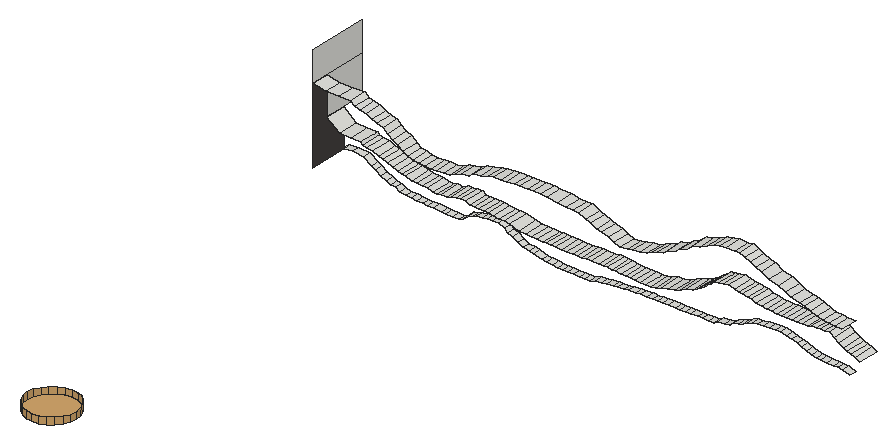
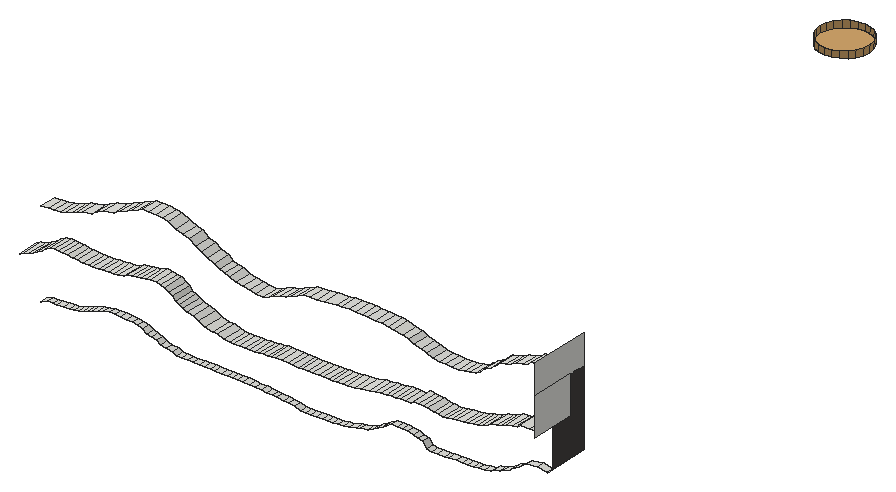
# SketchUp Ruby script. Lengths in inches.
U = 1.inch
M = Sketchup.active_model
def pt(a) = Geom::Point3d.new(a.map { |v| v * U })
def face(e, loops, mat)
  f = e.add_face(loops[0].map { |a| pt(a) })
  loops[1..].each { |l| e.add_face(l.map { |a| pt(a) }).erase! }
  f.material = f.back_material = mat if mat
  f
end
# faces: each face lists its corners as indices into pts; further lists are holes
def faces(e, pts, list, mat = nil) = list.each { |f| face(e, (f[0].is_a?(Array) ? f : [f]).map { |l| l.map { |i| pts[i] } }, mat) }
# xy, xz, yz: faces in a plane at the given z, y or x. An outline is a flat list of corners, or four numbers for a rectangle; further outlines are holes
def ring(l) = l.size == 4 ? [[l[0], l[1]], [l[2], l[1]], [l[2], l[3]], [l[0], l[3]]] : l.each_slice(2).to_a
def flat(e, list, mat, &to3) = list.each { |f| face(e, (f[0].is_a?(Array) ? f : [f]).map { |l| ring(l).map { |u, v| to3.(u, v) } }, mat) }
def xy(e, z, list, mat = nil) = flat(e, list, mat) { |x, y| [x, y, z] }
def xz(e, y, list, mat = nil) = flat(e, list, mat) { |x, z| [x, y, z] }
def yz(e, x, list, mat = nil) = flat(e, list, mat) { |y, z| [x, y, z] }
def lines(e, pts, list) = list.each { |a, b| e.add_line(pt(pts[a]), pt(pts[b])) }
# prism: a flat outline (further loops are holes) pulled along v
def prism(e, loops, v, mat = nil)
  f = face(e, loops, mat); d = Geom::Vector3d.new(v.map { |x| x * U })
  f.pushpull(f.normal.samedirection?(d) ? d.length : -d.length)
end
def box(e, o, s, mat = nil) = prism(e, [[o, [o[0] + s[0], o[1], o[2]], [o[0] + s[0], o[1] + s[1], o[2]], [o[0], o[1] + s[1], o[2]]]], [0, 0, s[2]], mat)
def at(x, y, z, deg = 0) = Geom::Transformation.translation(pt([x, y, z])) * Geom::Transformation.rotation(ORIGIN, Z_AXIS, deg.degrees)
def axes(o, x, y, z) = Geom::Transformation.new([*x, 0, *y, 0, *z, 0, *pt(o).to_a, 1])
def part(name) = M.definitions.add(name)
# library, detail: a bought-in or finely detailed component or shape, given as its bounding box
def library(name, o, s) = part(name).tap { |d| box(d.entities, o, s) }
def detail(e, o, s) = box(e.add_group.entities, o, s)
def put(e, d, t, mat = nil) = e.add_instance(d, t).tap { |i| i.material = mat if mat }
def group(e, t, mat = nil) = e.add_group.tap { |g| g.transformation = t; g.material = mat if mat }.entities
root = M.entities
M.materials.add("[Field Square Tile]").color = [211, 167, 108]
M.materials.add("[Granite Tile]1").color = [68, 65, 63]
xy(root,237.65,[[2918.33,2401.37,2919.02,2402.3],[2919.02,2401.37,2919.64,2402.3]])
xy(root,238.33,[[2927.43,2401.37,2927.98,2402.3],[2927.98,2401.37,2928.66,2402.3]])
xy(root,238.34,[[2929.34,2401.37,2930.27,2402.3],[2930.27,2401.37,2930.76,2402.3],[2930.76,2401.37,2931.52,2402.3],[2931.52,2401.37,2932.15,2402.3],[2932.15,2401.37,2932.9,2402.3],
  [2932.9,2401.37,2933.52,2402.3],[2933.52,2401.37,2934.29,2402.3],[2934.29,2401.37,2934.91,2402.3]])
xy(root,241.52,[[2889.03,2396.68,2889.09,2402.3]])
xy(root,241.68,[[2919.53,2398.8,2920.12,2401.37]])
xy(root,241.75,[[2921.88,2398.8,2922.75,2401.37],[2922.75,2398.8,2923.37,2401.37],[2923.37,2398.8,2923.88,2401.37]])
xy(root,250.6875,[[2909.35,2327.89,2908.56,2328,2907.82,2328.3,2907.18,2328.79,2906.7,2329.43,2906.39,2330.16,2906.29,2330.96,2906.39,2331.75,2906.7,2332.49,2907.18,2333.12,2907.82,2333.61,2908.56,2333.91,2909.35,2334.02,2910.14,2333.91,2910.88,2333.61,2911.51,2333.12,2912,2332.49,2912.31,2331.75,2912.41,2330.96,2912.31,2330.16,2912,2329.43,2911.51,2328.79,2910.88,2328.3,2910.14,2328]],"[Field Square Tile]")
xz(root,2396.68,[[2889.03,241.52,2889.09,251.5]])
yz(root,2889.09,[[2398.8,246.2,2404.3,250.88],[2396.68,250.88,2404.3,254.5]])
yz(root,2889.09,[[2396.68,241.52,2401.37,241.52,2401.37,246.2,2398.8,246.2,2398.8,250.88,2396.68,250.88]],"[Granite Tile]1")
p = [[2919.64,2401.37,237.65],[2919.64,2402.3,237.65],[2920.31,2402.3,237.89],[2920.31,2401.37,237.89],[2914.97,2401.37,237.76],[2914.97,2402.3,237.76],
  [2915.68,2402.3,237.71],[2915.68,2401.37,237.71],[2916.29,2402.3,237.68],[2916.29,2401.37,237.68],[2916.89,2402.3,237.67],[2916.89,2401.37,237.67],
  [2917.64,2402.3,237.66],[2917.64,2401.37,237.66],[2918.33,2402.3,237.65],[2918.33,2401.37,237.65],[2913.62,2401.37,237.9],[2913.62,2402.3,237.9],
  [2914.28,2402.3,237.82],[2914.28,2401.37,237.82],[2912.68,2401.37,238.21],[2912.68,2402.3,238.21],[2921.07,2402.3,237.94],[2921.07,2401.37,237.94],
  [2921.6875,2402.3,237.98],[2921.6875,2401.37,237.98],[2922.54,2402.3,238.1],[2922.54,2401.37,238.1],[2923.09,2402.3,238.13],[2923.09,2401.37,238.13],
  [2923.85,2402.3,238.15],[2923.85,2401.37,238.15],[2912.21,2401.37,238.31],[2912.21,2402.3,238.31],[2924.48,2402.3,238.26],[2924.48,2401.37,238.26],
  [2911.3,2401.37,238.43],[2911.3,2402.3,238.43],[2925.23,2402.3,238.28],[2925.23,2401.37,238.28],[2925.86,2402.3,238.3],[2925.86,2401.37,238.3],
  [2926.71,2402.3,238.32],[2926.71,2401.37,238.32],[2927.43,2402.3,238.33],[2927.43,2401.37,238.33],[2928.66,2401.37,238.33],[2928.66,2402.3,238.33],
  [2929.34,2402.3,238.34],[2929.34,2401.37,238.34],[2934.91,2401.37,238.34],[2934.91,2402.3,238.34],[2935.42,2402.3,238.59],[2935.42,2401.37,238.59],
  [2910.65,2401.37,238.74],[2910.65,2402.3,238.74],[2950.94,2401.37,238.78],[2950.94,2402.3,238.78],[2951.72,2402.3,238.43],[2951.72,2401.37,238.43],
  [2936.24,2402.3,238.72],[2936.24,2401.37,238.72],[2910.07,2401.37,239.11],[2910.07,2402.3,239.11],[2936.93,2402.3,238.86],[2936.93,2401.37,238.86],
  [2900.28,2401.37,238.92],[2900.28,2402.3,238.92],[2901.32,2402.3,238.82],[2901.32,2401.37,238.82],[2901.83,2402.3,238.8],[2901.83,2401.37,238.8],
  [2902.7,2402.3,238.79],[2902.7,2401.37,238.79],[2903.44,2402.3,238.77],[2903.44,2401.37,238.77],[2903.97,2402.3,238.9375],[2903.97,2401.37,238.9375],
  [2948.22,2401.37,238.875],[2948.22,2402.3,238.875],[2948.97,2402.3,238.83],[2948.97,2401.37,238.83],[2949.73,2402.3,238.8],[2949.73,2401.37,238.8],
  [2950.27,2402.3,238.79],[2950.27,2401.37,238.79],[2898.19,2401.37,238.97],[2898.19,2402.3,238.97],[2898.89,2402.3,238.94],[2898.89,2401.37,238.94],
  [2899.59,2402.3,238.93],[2899.59,2401.37,238.93],[2904.53,2402.3,239.55],[2904.53,2401.37,239.55],[2937.44,2402.3,239.18],[2937.44,2401.37,239.18],
  [2947.07,2401.37,239.04],[2947.07,2402.3,239.04],[2947.65,2402.3,238.94],[2947.65,2401.37,238.94],[2896.82,2401.37,239.09],[2896.82,2402.3,239.09],
  [2897.51,2402.3,239.03],[2897.51,2401.37,239.03],[2946.41,2401.37,239.29],[2946.41,2402.3,239.29],[2896.04,2401.37,239.19],[2896.04,2402.3,239.19],
  [2909.49,2401.37,239.38],[2909.49,2402.3,239.38],[2895.53,2401.37,239.52],[2895.53,2402.3,239.52],[2938.03,2402.3,239.35],[2938.03,2401.37,239.35],
  [2945.83,2401.37,239.53],[2945.83,2402.3,239.53],[2909.03,2401.37,239.71],[2909.03,2402.3,239.71],[2938.59,2402.3,239.52],[2938.59,2401.37,239.52],
  [2894.97,2401.37,239.64],[2894.97,2402.3,239.64],[2939.14,2402.3,239.85],[2939.14,2401.37,239.85],[2945.3,2401.37,239.7],[2945.3,2402.3,239.7],
  [2894.52,2401.37,239.86],[2894.52,2402.3,239.86],[2905.11,2402.3,239.69],[2905.11,2401.37,239.69],[2905.66,2402.3,239.88],[2905.66,2401.37,239.88],
  [2908.33,2401.37,240.11],[2908.33,2402.3,240.11],[2944.61,2401.37,239.92],[2944.61,2402.3,239.92],[2939.78,2402.3,240.03],[2939.78,2401.37,240.03],
  [2893.73,2401.37,240.2],[2893.73,2402.3,240.2],[2906.39,2402.3,239.99],[2906.39,2401.37,239.99],[2943.98,2401.37,240.11],[2943.98,2402.3,240.11],
  [2906.98,2402.3,240.05],[2906.98,2401.37,240.05],[2907.64,2402.3,240.09],[2907.64,2401.37,240.09],[2940.4375,2402.3,240.12],[2940.4375,2401.37,240.12],
  [2941.11,2402.3,240.19],[2941.11,2401.37,240.19],[2943.2,2401.37,240.27],[2943.2,2402.3,240.27],[2893.13,2401.37,240.59],[2893.13,2402.3,240.59],
  [2941.875,2402.3,240.23],[2941.875,2401.37,240.23],[2942.58,2402.3,240.25],[2942.58,2401.37,240.25],[2892.59,2401.37,240.85],[2892.59,2402.3,240.85],
  [2891.57,2401.37,241.55],[2891.57,2402.3,241.55],[2925.51,2398.8,241.57],[2925.51,2401.37,241.57],[2926.05,2401.37,241.53],[2926.05,2398.8,241.53],
  [2926.67,2401.37,241.51],[2926.67,2398.8,241.51],[2927.22,2401.37,241.49],[2927.22,2398.8,241.49],[2927.92,2401.37,241.48],[2927.92,2398.8,241.48],
  [2928.58,2401.37,241.47],[2928.58,2398.8,241.47],[2929.15,2401.37,241.46],[2929.15,2398.8,241.46],[2929.86,2401.37,241.6],[2929.86,2398.8,241.6],
  [2889.09,2401.37,241.52],[2889.09,2402.3,241.52],[2890.3,2402.3,241.69],[2890.3,2401.37,241.69],[2924.9,2398.8,241.66],[2924.9,2401.37,241.66],
  [2930.59,2401.37,241.85],[2930.59,2398.8,241.85],[2915.87,2398.8,241.75],[2915.87,2401.37,241.75],[2916.32,2401.37,241.74],[2916.32,2398.8,241.74],
  [2916.87,2401.37,241.72],[2916.87,2398.8,241.72],[2917.5,2401.37,241.71],[2917.5,2398.8,241.71],[2918.13,2401.37,241.7],[2918.13,2398.8,241.7],
  [2918.86,2401.37,241.69],[2918.86,2398.8,241.69],[2919.53,2401.37,241.68],[2919.53,2398.8,241.68],[2920.12,2398.8,241.68],[2920.12,2401.37,241.68],
  [2920.61,2401.37,241.67],[2920.61,2398.8,241.67],[2921.3125,2401.37,241.74],[2921.3125,2398.8,241.74],[2921.88,2401.37,241.75],[2921.88,2398.8,241.75],
  [2923.88,2398.8,241.75],[2923.88,2401.37,241.75],[2924.37,2401.37,241.67],[2924.37,2398.8,241.67],[2913.68,2398.8,241.89],[2913.68,2401.37,241.89],
  [2914.5,2401.37,241.83],[2914.5,2398.8,241.83],[2915.1,2401.37,241.78],[2915.1,2398.8,241.78],[2931.26,2401.37,241.91],[2931.26,2398.8,241.91],
  [2912.91,2398.8,241.96],[2912.91,2401.37,241.96],[2932.16,2401.37,242.1],[2932.16,2398.8,242.1],[2911.74,2398.8,242.24],[2911.74,2401.37,242.24],
  [2932.93,2401.37,242.46],[2932.93,2398.8,242.46],[2911.07,2398.8,242.34],[2911.07,2401.37,242.34],[2954.54,2398.8,242.51],[2954.54,2401.37,242.51],
  [2955.05,2401.37,242.21],[2955.05,2398.8,242.21],[2910.41,2398.8,242.38],[2910.41,2401.37,242.38],[2909.75,2398.8,242.48],[2909.75,2401.37,242.48],
  [2901.57,2398.8,242.68],[2901.57,2401.37,242.68],[2902.24,2401.37,242.51],[2902.24,2398.8,242.51],[2902.76,2401.37,242.46],[2902.76,2398.8,242.46],
  [2903.3,2401.37,242.58],[2903.3,2398.8,242.58],[2909.11,2398.8,242.57],[2909.11,2401.37,242.57],[2933.63,2401.37,242.78],[2933.63,2398.8,242.78],
  [2953.95,2398.8,242.68],[2953.95,2401.37,242.68],[2903.93,2401.37,242.57],[2903.93,2398.8,242.57],[2904.56,2401.37,242.81],[2904.56,2398.8,242.81],
  [2906.33,2398.8,242.92],[2906.33,2401.37,242.92],[2906.76,2401.37,242.625],[2906.76,2398.8,242.625],[2907.37,2401.37,242.65],[2907.37,2398.8,242.65],
  [2907.92,2401.37,242.62],[2907.92,2398.8,242.62],[2908.55,2401.37,242.58],[2908.55,2398.8,242.58],[2900.22,2398.8,242.78],[2900.22,2401.37,242.78],
  [2901.03,2401.37,242.73],[2901.03,2398.8,242.73],[2953.45,2398.8,242.875],[2953.45,2401.37,242.875],[2898.92,2398.8,243.06],[2898.92,2401.37,243.06],
  [2899.64,2401.37,242.85],[2899.64,2398.8,242.85],[2905.13,2401.37,242.86],[2905.13,2398.8,242.86],[2934.4,2401.37,242.97],[2934.4,2398.8,242.97],
  [2905.69,2401.37,242.89],[2905.69,2398.8,242.89],[2953.06,2398.8,243.09],[2953.06,2401.37,243.09],[2934.93,2401.37,243.23],[2934.93,2398.8,243.23],
  [2897.85,2398.8,243.3],[2897.85,2401.37,243.3],[2898.4375,2401.37,243.14],[2898.4375,2398.8,243.14],[2952.45,2398.8,243.43],[2952.45,2401.37,243.43],
  [2935.33,2401.37,243.48],[2935.33,2398.8,243.48],[2897.21,2398.8,243.48],[2897.21,2401.37,243.48],[2951.91,2398.8,243.8],[2951.91,2401.37,243.8],
  [2896.69,2398.8,243.79],[2896.69,2401.37,243.79],[2935.85,2401.37,243.72],[2935.85,2398.8,243.72],[2936.1875,2401.37,244.12],[2936.1875,2398.8,244.12],
  [2896.03,2398.8,243.95],[2896.03,2401.37,243.95],[2951.31,2398.8,244.18],[2951.31,2401.37,244.18],[2895.51,2398.8,244.11],[2895.51,2401.37,244.11],
  [2944.13,2398.8,243.99],[2944.13,2401.37,243.99],[2944.85,2401.37,243.95],[2944.85,2398.8,243.95],[2945.35,2401.37,243.93],[2945.35,2398.8,243.93],
  [2946.04,2401.37,243.91],[2946.04,2398.8,243.91],[2946.61,2401.37,243.89],[2946.61,2398.8,243.89],[2947.31,2401.37,243.88],[2947.31,2398.8,243.88],
  [2947.96,2401.37,243.94],[2947.96,2398.8,243.94],[2948.6,2401.37,243.95],[2948.6,2398.8,243.95],[2949.16,2401.37,244.1],[2949.16,2398.8,244.1],
  [2942.95,2398.8,244.11],[2942.95,2401.37,244.11],[2943.51,2401.37,244.04],[2943.51,2398.8,244.04],[2894.84,2398.8,244.41],[2894.84,2401.37,244.41],
  [2936.66,2401.37,244.39],[2936.66,2398.8,244.39],[2942.2,2398.8,244.25],[2942.2,2401.37,244.25],[2949.79,2401.37,244.13],[2949.79,2398.8,244.13],
  [2950.27,2401.37,244.15],[2950.27,2398.8,244.15],[2950.79,2401.37,244.17],[2950.79,2398.8,244.17],[2941.74,2398.8,244.51],[2941.74,2401.37,244.51],
  [2894.08,2398.8,244.54],[2894.08,2401.37,244.54],[2937.14,2401.37,244.73],[2937.14,2398.8,244.73],[2893.52,2398.8,244.61],[2893.52,2401.37,244.61],
  [2940.59,2398.8,244.67],[2940.59,2401.37,244.67],[2941.2,2401.37,244.55],[2941.2,2398.8,244.55],[2893.3,2398.8,244.92],[2893.3,2401.37,244.92],
  [2937.625,2401.37,244.87],[2937.625,2398.8,244.87],[2939.54,2398.8,244.81],[2939.54,2401.37,244.81],[2940.11,2401.37,244.7],[2940.11,2398.8,244.7],
  [2938.89,2398.8,245.01],[2938.89,2401.37,245.01],[2890.66,2398.8,244.96],[2890.66,2401.37,244.96],[2892.05,2401.37,244.9375],[2892.05,2398.8,244.9375],
  [2938.21,2401.37,244.95],[2938.21,2398.8,244.95],[2889.09,2398.8,246.2],[2889.09,2401.37,246.2],[2926.34,2396.68,246.35],[2926.34,2398.8,246.35],
  [2927.11,2398.8,246.05],[2927.11,2396.68,246.05],[2928.01,2398.8,246.13],[2928.01,2396.68,246.13],[2928.72,2398.8,246.29],[2928.72,2396.68,246.29],
  [2929.52,2398.8,246.41],[2929.52,2396.68,246.41],[2925.73,2396.68,246.66],[2925.73,2398.8,246.66],[2930.43,2398.8,246.55],[2930.43,2396.68,246.55],
  [2902.15,2396.68,246.62],[2902.15,2398.8,246.62],[2902.89,2398.8,246.54],[2902.89,2396.68,246.54],[2903.67,2398.8,246.51],[2903.67,2396.68,246.51],
  [2904.45,2398.8,246.58],[2904.45,2396.68,246.58],[2953.64,2396.68,246.59],[2953.64,2398.8,246.59],[2954.53,2398.8,246.55],[2954.53,2396.68,246.55],
  [2901.49,2396.68,246.73],[2901.49,2398.8,246.73],[2905.25,2398.8,246.59],[2905.25,2396.68,246.59],[2906.05,2398.8,246.69],[2906.05,2396.68,246.69],
  [2931.16,2398.8,246.92],[2931.16,2396.68,246.92],[2952.93,2396.68,246.66],[2952.93,2398.8,246.66],[2900.77,2396.68,246.88],[2900.77,2398.8,246.88],
  [2906.76,2398.8,247.03],[2906.76,2396.68,247.03],[2924.875,2396.68,246.94],[2924.875,2398.8,246.94],[2952.14,2396.68,246.75],[2952.14,2398.8,246.75],
  [2951.45,2396.68,246.95],[2951.45,2398.8,246.95],[2900.22,2396.68,247.25],[2900.22,2398.8,247.25],[2924.19,2396.68,247.08],[2924.19,2398.8,247.08],
  [2931.77,2398.8,247.12],[2931.77,2396.68,247.12],[2907.45,2398.8,247.2],[2907.45,2396.68,247.2],[2950.64,2396.68,247.25],[2950.64,2398.8,247.25],
  [2923.51,2396.68,247.46],[2923.51,2398.8,247.46],[2932.45,2398.8,247.31],[2932.45,2396.68,247.31],[2908.42,2398.8,247.39],[2908.42,2396.68,247.39],
  [2949.96,2396.68,247.53],[2949.96,2398.8,247.53],[2899.58,2396.68,247.72],[2899.58,2398.8,247.72],[2933.02,2398.8,247.71],[2933.02,2396.68,247.71],
  [2909.05,2398.8,247.78],[2909.05,2396.68,247.78],[2922.88,2396.68,247.66],[2922.88,2398.8,247.66],[2949.38,2396.68,247.66],[2949.38,2398.8,247.66],
  [2898.93,2396.68,248.07],[2898.93,2398.8,248.07],[2922.04,2396.68,248.08],[2922.04,2398.8,248.08],[2933.95,2398.8,248.03],[2933.95,2396.68,248.03],
  [2948.25,2396.68,247.9],[2948.25,2398.8,247.9],[2909.83,2398.8,247.89],[2909.83,2396.68,247.89],[2910.83,2398.8,248.18],[2910.83,2396.68,248.18],
  [2947.65,2396.68,248.26],[2947.65,2398.8,248.26],[2934.66,2398.8,248.46],[2934.66,2396.68,248.46],[2898.3,2396.68,248.51],[2898.3,2398.8,248.51],
  [2920.42,2396.68,248.15],[2920.42,2398.8,248.15],[2921.24,2398.8,248.11],[2921.24,2396.68,248.11],[2911.47,2398.8,248.29],[2911.47,2396.68,248.29],
  [2919.39,2396.68,248.28],[2919.39,2398.8,248.28],[2912.36,2398.8,248.35],[2912.36,2396.68,248.35],[2917.99,2396.68,248.39],[2917.99,2398.8,248.39],
  [2946.74,2396.68,248.69],[2946.74,2398.8,248.69],[2913.09,2398.8,248.4],[2913.09,2396.68,248.4],[2914.08,2398.8,248.4375],[2914.08,2396.68,248.4375],
  [2914.74,2398.8,248.46],[2914.74,2396.68,248.46],[2917.26,2396.68,248.49],[2917.26,2398.8,248.49],[2897.81,2396.68,249.01],[2897.81,2398.8,249.01],
  [2915.63,2398.8,248.47],[2915.63,2396.68,248.47],[2916.37,2398.8,248.48],[2916.37,2396.68,248.48],[2935.44,2398.8,248.82],[2935.44,2396.68,248.82],
  [2945.52,2396.68,248.95],[2945.52,2398.8,248.95],[2936.16,2398.8,249.37],[2936.16,2396.68,249.37],[2944.63,2396.68,249.46],[2944.63,2398.8,249.46],
  [2897.04,2396.68,249.2],[2897.04,2398.8,249.2],[2896.37,2396.68,249.41],[2896.37,2398.8,249.41],[2895.7,2396.68,249.8],[2895.7,2398.8,249.8],
  [2936.95,2398.8,249.5625],[2936.95,2396.68,249.5625],[2943.87,2396.68,249.68],[2943.87,2398.8,249.68],[2937.85,2398.8,249.9],[2937.85,2396.68,249.9],
  [2943.21,2396.68,250.0625],[2943.21,2398.8,250.0625],[2894.9,2396.68,249.97],[2894.9,2398.8,249.97],[2938.77,2398.8,250.35],[2938.77,2396.68,250.35],
  [2894.29,2396.68,250.15],[2894.29,2398.8,250.15],[2893.76,2396.68,250.55],[2893.76,2398.8,250.55],[2942.52,2396.68,250.32],[2942.52,2398.8,250.32],
  [2939.43,2398.8,250.49],[2939.43,2396.68,250.49],[2941.9,2396.68,250.61],[2941.9,2398.8,250.61],[2889.09,2396.68,250.88],[2889.09,2398.8,250.88],
  [2890.68,2398.8,250.53],[2890.68,2396.68,250.53],[2892.3,2398.8,250.54],[2892.3,2396.68,250.54],[2940.24,2398.8,250.6],[2940.24,2396.68,250.6],
  [2941.26,2398.8,250.58],[2941.26,2396.68,250.58],[2909.35,2327.89,251.5],[2908.56,2328,251.5],[2908.56,2328,250.6875],[2909.35,2327.89,250.6875],
  [2910.14,2328,251.5],[2910.14,2328,250.6875],[2907.82,2328.3,251.5],[2907.82,2328.3,250.6875],[2910.88,2328.3,251.5],[2910.88,2328.3,250.6875],
  [2907.18,2328.79,251.5],[2907.18,2328.79,250.6875],[2911.51,2328.79,251.5],[2911.51,2328.79,250.6875],[2906.7,2329.43,251.5],[2906.7,2329.43,250.6875],
  [2912,2329.43,251.5],[2912,2329.43,250.6875],[2906.39,2330.16,251.5],[2906.39,2330.16,250.6875],[2912.31,2330.16,251.5],[2912.31,2330.16,250.6875],
  [2906.29,2330.96,251.5],[2906.29,2330.96,250.6875],[2912.41,2330.96,251.5],[2912.41,2330.96,250.6875],[2906.39,2331.75,251.5],[2906.39,2331.75,250.6875],
  [2912.31,2331.75,251.5],[2912.31,2331.75,250.6875],[2906.7,2332.49,251.5],[2906.7,2332.49,250.6875],[2912,2332.49,251.5],[2912,2332.49,250.6875],
  [2907.18,2333.12,251.5],[2907.18,2333.12,250.6875],[2911.51,2333.12,251.5],[2911.51,2333.12,250.6875],[2907.82,2333.61,251.5],[2907.82,2333.61,250.6875],
  [2910.88,2333.61,251.5],[2910.88,2333.61,250.6875],[2908.56,2333.91,251.5],[2908.56,2333.91,250.6875],[2910.14,2333.91,251.5],[2910.14,2333.91,250.6875],
  [2909.35,2334.02,251.5],[2909.35,2334.02,250.6875]]
faces(root,p,[[0,1,2,3],[4,5,6,7],[7,6,8,9],[9,8,10,11],[11,10,12,13],[13,12,14,15],[16,17,18,19],[19,18,5,4],
  [20,21,17,16],[3,2,22,23],[23,22,24,25],[25,24,26,27],[27,26,28,29],[29,28,30,31],[32,33,21,20],[31,30,34,35],
  [36,37,33,32],[35,34,38,39],[39,38,40,41],[41,40,42,43],[43,42,44,45],[46,47,48,49],[50,51,52,53],[54,55,37,36],
  [56,57,58,59],[53,52,60,61],[62,63,55,54],[61,60,64,65],[66,67,68,69],[69,68,70,71],[71,70,72,73],[73,72,74,75],
  [75,74,76,77],[78,79,80,81],[81,80,82,83],[83,82,84,85],[85,84,57,56],[86,87,88,89],[89,88,90,91],[91,90,67,66],
  [77,76,92,93],[65,64,94,95],[96,97,98,99],[99,98,79,78],[100,101,102,103],[103,102,87,86],[104,105,97,96],[106,107,101,100],
  [108,109,63,62],[110,111,107,106],[95,94,112,113],[114,115,105,104],[116,117,109,108],[113,112,118,119],[120,121,111,110],[119,118,122,123],
  [124,125,115,114],[126,127,121,120],[93,92,128,129],[129,128,130,131],[132,133,117,116],[134,135,125,124],[123,122,136,137],[138,139,127,126],
  [131,130,140,141],[142,143,135,134],[141,140,144,145],[145,144,146,147],[137,136,148,149],[147,146,133,132],[149,148,150,151],[152,153,143,142],
  [154,155,139,138],[151,150,156,157],[157,156,158,159],[159,158,153,152],[160,161,155,154],[162,163,161,160],[164,165,166,167],[167,166,168,169],
  [169,168,170,171],[171,170,172,173],[173,172,174,175],[175,174,176,177],[177,176,178,179],[180,181,182,183],[184,185,165,164],[179,178,186,187],
  [183,182,163,162],[188,189,190,191],[191,190,192,193],[193,192,194,195],[195,194,196,197],[197,196,198,199],[199,198,200,201],[202,203,204,205],
  [205,204,206,207],[207,206,208,209],[210,211,212,213],[213,212,185,184],[214,215,216,217],[217,216,218,219],[219,218,189,188],[187,186,220,221],
  [222,223,215,214],[221,220,224,225],[226,227,223,222],[225,224,228,229],[230,231,227,226],[232,233,234,235],[236,237,231,230],[238,239,237,236],
  [240,241,242,243],[243,242,244,245],[245,244,246,247],[248,249,239,238],[229,228,250,251],[252,253,233,232],[247,246,254,255],[255,254,256,257],
  [258,259,260,261],[261,260,262,263],[263,262,264,265],[265,264,266,267],[267,266,249,248],[268,269,270,271],[271,270,241,240],[272,273,253,252],
  [274,275,276,277],[277,276,269,268],[257,256,278,279],[251,250,280,281],[279,278,282,283],[283,282,259,258],[284,285,273,272],[281,280,286,287],
  [288,289,290,291],[291,290,275,274],[292,293,285,284],[287,286,294,295],[296,297,289,288],[298,299,293,292],[300,301,297,296],[295,294,302,303],
  [303,302,304,305],[306,307,301,300],[308,309,299,298],[310,311,307,306],[312,313,314,315],[315,314,316,317],[317,316,318,319],[319,318,320,321],
  [321,320,322,323],[323,322,324,325],[325,324,326,327],[327,326,328,329],[330,331,332,333],[333,332,313,312],[334,335,311,310],[305,304,336,337],
  [338,339,331,330],[329,328,340,341],[341,340,342,343],[343,342,344,345],[345,344,309,308],[346,347,339,338],[348,349,335,334],[337,336,350,351],
  [352,353,349,348],[354,355,356,357],[357,356,347,346],[358,359,353,352],[351,350,360,361],[362,363,364,365],[365,364,355,354],[366,367,363,362],
  [368,369,370,371],[371,370,359,358],[361,360,372,373],[373,372,367,366],[374,375,369,368],[376,377,378,379],[379,378,380,381],[381,380,382,383],
  [383,382,384,385],[386,387,377,376],[385,384,388,389],[390,391,392,393],[393,392,394,395],[395,394,396,397],[398,399,400,401],[402,403,391,390],
  [397,396,404,405],[405,404,406,407],[389,388,408,409],[410,411,399,398],[412,413,403,402],[407,406,414,415],[416,417,387,386],[418,419,411,410],
  [420,421,419,418],[422,423,413,412],[424,425,417,416],[409,408,426,427],[415,414,428,429],[430,431,421,420],[432,433,425,424],[427,426,434,435],
  [429,428,436,437],[438,439,431,430],[440,441,423,422],[435,434,442,443],[437,436,444,445],[446,447,433,432],[448,449,439,438],[450,451,441,440],
  [452,453,447,446],[443,442,454,455],[456,457,449,448],[445,444,458,459],[459,458,460,461],[462,463,457,456],[455,454,464,465],[466,467,451,450],
  [468,469,470,471],[471,470,453,452],[461,460,472,473],[474,475,469,468],[473,472,476,477],[478,479,475,474],[480,481,463,462],[477,476,482,483],
  [483,482,484,485],[485,484,486,487],[488,489,479,478],[490,491,467,466],[487,486,492,493],[493,492,494,495],[495,494,489,488],[465,464,496,497],
  [498,499,481,480],[497,496,500,501],[502,503,499,498],[504,505,491,490],[506,507,505,504],[508,509,507,506],[501,500,510,511],[512,513,503,502],
  [511,510,514,515],[516,517,513,512],[518,519,509,508],[515,514,520,521],[522,523,519,518],[524,525,523,522],[526,527,517,516],[521,520,528,529],
  [530,531,527,526],[532,533,534,535],[535,534,536,537],[537,536,525,524],[529,528,538,539],[539,538,540,541],[541,540,531,530]])
faces(root,p,[[542,543,544,545],[546,542,545,547],[543,548,549,544],[550,546,547,551],[548,552,553,549],[554,550,551,555],[552,556,557,553],[558,554,555,559],
  [556,560,561,557],[562,558,559,563],[560,564,565,561],[566,562,563,567],[564,568,569,565],[570,566,567,571],[568,572,573,569],[574,570,571,575],
  [572,576,577,573],[578,574,575,579],[576,580,581,577],[582,578,579,583],[580,584,585,581],[586,582,583,587],[584,588,589,585],[588,586,587,589]],"[Field Square Tile]")
